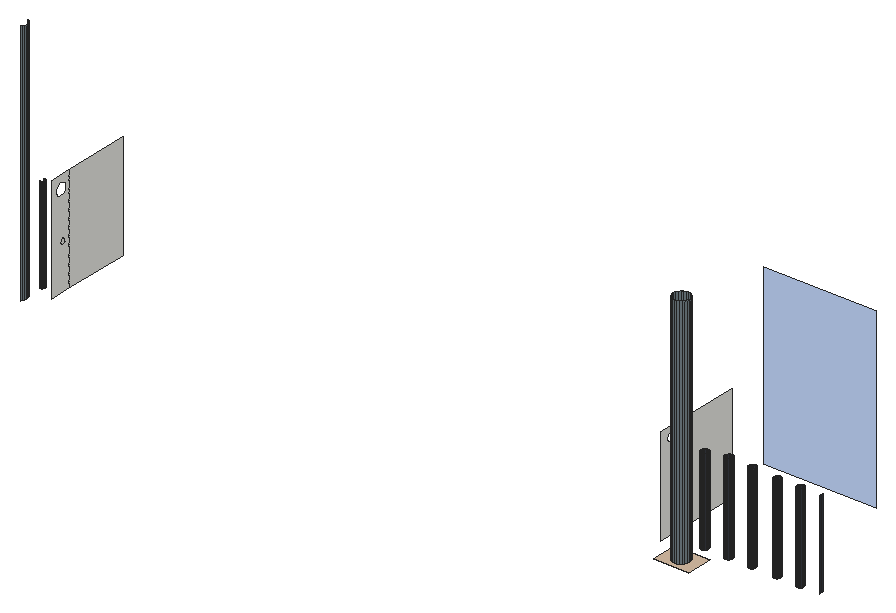
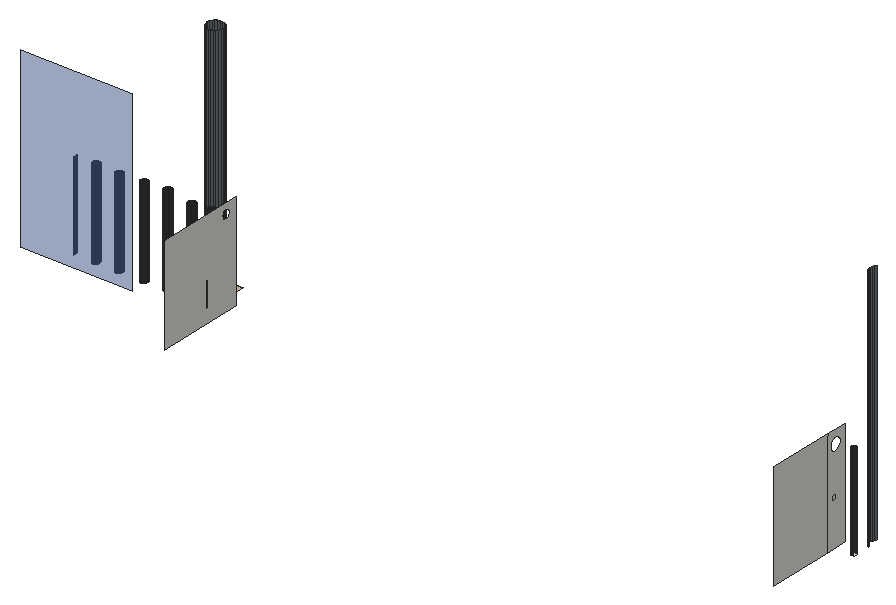
# SketchUp Ruby script. Lengths in inches.
U = 1.inch
M = Sketchup.active_model
def pt(a) = Geom::Point3d.new(a.map { |v| v * U })
def face(e, loops, mat)
  f = e.add_face(loops[0].map { |a| pt(a) })
  loops[1..].each { |l| e.add_face(l.map { |a| pt(a) }).erase! }
  f.material = f.back_material = mat if mat
  f
end
# faces: each face lists its corners as indices into pts; further lists are holes
def faces(e, pts, list, mat = nil) = list.each { |f| face(e, (f[0].is_a?(Array) ? f : [f]).map { |l| l.map { |i| pts[i] } }, mat) }
# xy, xz, yz: faces in a plane at the given z, y or x. An outline is a flat list of corners, or four numbers for a rectangle; further outlines are holes
def ring(l) = l.size == 4 ? [[l[0], l[1]], [l[2], l[1]], [l[2], l[3]], [l[0], l[3]]] : l.each_slice(2).to_a
def flat(e, list, mat, &to3) = list.each { |f| face(e, (f[0].is_a?(Array) ? f : [f]).map { |l| ring(l).map { |u, v| to3.(u, v) } }, mat) }
def xy(e, z, list, mat = nil) = flat(e, list, mat) { |x, y| [x, y, z] }
def xz(e, y, list, mat = nil) = flat(e, list, mat) { |x, z| [x, y, z] }
def yz(e, x, list, mat = nil) = flat(e, list, mat) { |y, z| [x, y, z] }
def lines(e, pts, list) = list.each { |a, b| e.add_line(pt(pts[a]), pt(pts[b])) }
# prism: a flat outline (further loops are holes) pulled along v
def prism(e, loops, v, mat = nil)
  f = face(e, loops, mat); d = Geom::Vector3d.new(v.map { |x| x * U })
  f.pushpull(f.normal.samedirection?(d) ? d.length : -d.length)
end
def box(e, o, s, mat = nil) = prism(e, [[o, [o[0] + s[0], o[1], o[2]], [o[0] + s[0], o[1] + s[1], o[2]], [o[0], o[1] + s[1], o[2]]]], [0, 0, s[2]], mat)
def at(x, y, z, deg = 0) = Geom::Transformation.translation(pt([x, y, z])) * Geom::Transformation.rotation(ORIGIN, Z_AXIS, deg.degrees)
def axes(o, x, y, z) = Geom::Transformation.new([*x, 0, *y, 0, *z, 0, *pt(o).to_a, 1])
def part(name) = M.definitions.add(name)
# library, detail: a bought-in or finely detailed component or shape, given as its bounding box
def library(name, o, s) = part(name).tap { |d| box(d.entities, o, s) }
def detail(e, o, s) = box(e.add_group.entities, o, s)
def put(e, d, t, mat = nil) = e.add_instance(d, t).tap { |i| i.material = mat if mat }
def group(e, t, mat = nil) = e.add_group.tap { |g| g.transformation = t; g.material = mat if mat }.entities
root = M.entities
M.materials.add("[Color M07]").color = [58, 58, 58]
M.materials.add("[Formica Laminate Dark]").color = [50, 53, 60]
M.materials.add("[Formica Laminate Light]").color = [213, 189, 164]
M.materials.add("[Formica Speckled Grey]").color = [112, 125, 132]
M.materials.add("[Translucent Glass Blue]").color = [85, 126, 201]
M.materials["[Translucent Glass Blue]"].alpha = 0.5
xy(root,272.93,[[302.73,84.01,302.14,84.08,301.6,84.31,301.14,84.67,300.78,85.13,300.55,85.67,300.48,86.26,300.55,86.84,300.78,87.38,301.14,87.85,301.6,88.21,302.14,88.43,302.73,88.51,303.31,88.43,303.85,88.21,304.32,87.85,304.67,87.38,304.9,86.84,304.98,86.26,304.9,85.67,304.67,85.13,304.32,84.67,303.85,84.31,303.31,84.08],[298.07,92.22,297.82,92.25,297.57,92.35,297.37,92.51,297.21,92.72,297.11,92.96,297.07,93.22,297.11,93.48,297.21,93.72,297.37,93.93,297.57,94.09,297.82,94.1875,298.07,94.22,298.33,94.1875,298.57,94.09,298.78,93.93,298.94,93.72,299.04,93.48,299.07,93.22,299.04,92.96,298.94,92.72,298.78,92.51,298.57,92.35,298.33,92.25],[303.57,92.22,303.32,92.25,303.07,92.35,302.87,92.51,302.71,92.72,302.61,92.96,302.57,93.22,302.61,93.48,302.71,93.72,302.87,93.93,303.07,94.09,303.32,94.1875,303.57,94.22,303.83,94.1875,304.07,94.09,304.28,93.93,304.44,93.72,304.54,93.48,304.57,93.22,304.54,92.96,304.44,92.72,304.28,92.51,304.07,92.35,303.83,92.25],[310.2,92.22,309.94,92.25,309.7,92.35,309.49,92.51,309.33,92.72,309.23,92.96,309.2,93.22,309.23,93.48,309.33,93.72,309.49,93.93,309.7,94.09,309.94,94.1875,310.2,94.22,310.46,94.1875,310.7,94.09,310.91,93.93,311.07,93.72,311.17,93.48,311.2,93.22,311.17,92.96,311.07,92.72,310.91,92.51,310.7,92.35,310.46,92.25],[316.7,92.22,316.44,92.25,316.2,92.35,315.99,92.51,315.83,92.72,315.73,92.96,315.7,93.22,315.73,93.48,315.83,93.72,315.99,93.93,316.2,94.09,316.44,94.1875,316.7,94.22,316.96,94.1875,317.2,94.09,317.41,93.93,317.57,93.72,317.67,93.48,317.7,93.22,317.67,92.96,317.57,92.72,317.41,92.51,317.2,92.35,316.96,92.25],
  [323.57,92.22,323.32,92.25,323.07,92.35,322.87,92.51,322.71,92.72,322.61,92.96,322.57,93.22,322.61,93.48,322.71,93.72,322.87,93.93,323.07,94.09,323.32,94.1875,323.57,94.22,323.83,94.1875,324.07,94.09,324.28,93.93,324.44,93.72,324.54,93.48,324.57,93.22,324.54,92.96,324.44,92.72,324.28,92.51,324.07,92.35,323.83,92.25],[329.95,92.22,329.69,92.25,329.45,92.35,329.24,92.51,329.08,92.72,328.98,92.96,328.95,93.22,328.98,93.48,329.08,93.72,329.24,93.93,329.45,94.09,329.69,94.1875,329.95,94.22,330.21,94.1875,330.45,94.09,330.66,93.93,330.82,93.72,330.92,93.48,330.95,93.22,330.92,92.96,330.82,92.72,330.66,92.51,330.45,92.35,330.21,92.25]])
xy(root,272.93,[[[298.18,82.54,307.63,89.73],[302.73,84.01,302.14,84.08,301.6,84.31,301.14,84.67,300.78,85.13,300.55,85.67,300.48,86.26,300.55,86.84,300.78,87.38,301.14,87.85,301.6,88.21,302.14,88.43,302.73,88.51,303.31,88.43,303.85,88.21,304.32,87.85,304.67,87.38,304.9,86.84,304.98,86.26,304.9,85.67,304.67,85.13,304.32,84.67,303.85,84.31,303.31,84.08]]],"[Formica Laminate Light]")
xy(root,273.71,[[121.84,91.87,121.66,91.89,121.5,91.96,121.36,92.07,121.25,92.21,121.18,92.38,121.15,92.56,121.18,92.73,121.25,92.9,121.36,93.04,121.5,93.15,121.66,93.22,121.84,93.24,122.02,93.22,122.1875,93.15,122.33,93.04,122.4375,92.9,122.51,92.73,122.53,92.56,122.51,92.38,122.4375,92.21,122.33,92.07,122.1875,91.96,122.02,91.89]])
xz(root,114.1,[[303.24,284.18,334.08,332.96]],"[Translucent Glass Blue]")
yz(root,126.66,[[[89.73,273.71,95.59,302.83],[92.96,297.54,93.42,297.6,93.84,297.77,94.2,298.05,94.48,298.41,94.65,298.84,94.71,299.29,94.65,299.74,94.48,300.16,94.2,300.53,93.84,300.8,93.42,300.98,92.96,301.04,92.51,300.98,92.09,300.8,91.73,300.53,91.45,300.16,91.27,299.74,91.21,299.29,91.27,298.84,91.45,298.41,91.73,298.05,92.09,297.77,92.51,297.6],[93.52,285.62,93.72,285.64,93.9,285.72,94.05,285.84,94.17,285.99,94.25,286.17,94.27,286.37,94.25,286.5625,94.17,286.74,94.05,286.9,93.9,287.02,93.72,287.09,93.52,287.12,93.33,287.09,93.15,287.02,92.99,286.9,92.875,286.74,92.8,286.5625,92.77,286.37,92.8,286.17,92.875,285.99,92.99,285.84,93.15,285.72,93.33,285.64]],[95.59,273.71,114.1,302.83],[93.52,285.62,93.72,285.64,93.9,285.72,94.05,285.84,94.17,285.99,94.25,286.17,94.27,286.37,94.25,286.5625,94.17,286.74,94.05,286.9,93.9,287.02,93.72,287.09,93.52,287.12,93.33,287.09,93.15,287.02,92.99,286.9,92.875,286.74,92.8,286.5625,92.77,286.37,92.8,286.17,92.875,285.99,92.99,285.84,93.15,285.72,93.33,285.64]])
yz(root,294.34,[[[89.73,272.93,114.1,299.8],[93.0625,295.87,92.74,295.91,92.4375,296.04,92.18,296.23,91.98,296.49,91.86,296.79,91.8125,297.12,91.86,297.44,91.98,297.74,92.18,298,92.4375,298.2,92.74,298.33,93.0625,298.37,93.39,298.33,93.6875,298.2,93.95,298,94.15,297.74,94.27,297.44,94.3125,297.12,94.27,296.79,94.15,296.49,93.95,296.23,93.6875,296.04,93.39,295.91]]])
p = [[302.14,84.08,272.93],[302.73,84.01,272.93],[302.73,84.01,337.71],[302.14,84.08,337.71],[303.31,84.08,272.93],[303.31,84.08,337.71],
  [301.6,84.31,272.93],[301.6,84.31,337.71],[303.85,84.31,272.93],[303.85,84.31,337.71],[301.14,84.67,272.93],[301.14,84.67,337.71],
  [304.32,84.67,272.93],[304.32,84.67,337.71],[300.78,85.13,272.93],[300.78,85.13,337.71],[304.67,85.13,272.93],[304.67,85.13,337.71],
  [300.55,85.67,272.93],[300.55,85.67,337.71],[304.9,85.67,272.93],[304.9,85.67,337.71],[300.48,86.26,272.93],[300.48,86.26,337.71],
  [304.98,86.26,272.93],[304.98,86.26,337.71],[300.55,86.84,272.93],[300.55,86.84,337.71],[304.9,86.84,272.93],[304.9,86.84,337.71],
  [300.78,87.38,272.93],[300.78,87.38,337.71],[304.67,87.38,272.93],[304.67,87.38,337.71],[301.14,87.85,272.93],[301.14,87.85,337.71],
  [304.32,87.85,272.93],[304.32,87.85,337.71],[301.6,88.21,272.93],[301.6,88.21,337.71],[303.85,88.21,272.93],[303.85,88.21,337.71],
  [302.14,88.43,272.93],[302.14,88.43,337.71],[303.31,88.43,272.93],[303.31,88.43,337.71],[302.73,88.51,272.93],[302.73,88.51,337.71],
  [297.82,92.25,272.93],[298.07,92.22,272.93],[298.07,92.22,297.05],[297.82,92.25,297.05],[298.33,92.25,272.93],[298.33,92.25,297.05],
  [303.32,92.25,272.93],[303.57,92.22,272.93],[303.57,92.22,296.68],[303.32,92.25,296.68],[303.83,92.25,272.93],[303.83,92.25,296.68],
  [309.94,92.25,272.93],[310.2,92.22,272.93],[310.2,92.22,297.74],[309.94,92.25,297.74],[310.46,92.25,272.93],[310.46,92.25,297.74],
  [316.44,92.25,272.93],[316.7,92.22,272.93],[316.7,92.22,297.44],[316.44,92.25,297.44],[316.96,92.25,272.93],[316.96,92.25,297.44],
  [323.32,92.25,272.93],[323.57,92.22,272.93],[323.57,92.22,297.05],[323.32,92.25,297.05],[323.83,92.25,272.93],[323.83,92.25,297.05],
  [329.69,92.25,272.93],[329.95,92.22,272.93],[329.95,92.22,297.18],[329.69,92.25,297.18],[330.21,92.25,272.93],[330.21,92.25,297.18],
  [297.57,92.35,272.93],[297.57,92.35,297.05],[298.57,92.35,272.93],[298.57,92.35,297.05],[303.07,92.35,272.93],[303.07,92.35,296.68],
  [304.07,92.35,272.93],[304.07,92.35,296.68],[309.7,92.35,272.93],[309.7,92.35,297.74],[310.7,92.35,272.93],[310.7,92.35,297.74],
  [316.2,92.35,272.93],[316.2,92.35,297.44],[317.2,92.35,272.93],[317.2,92.35,297.44],[323.07,92.35,272.93],[323.07,92.35,297.05],
  [324.07,92.35,272.93],[324.07,92.35,297.05],[329.45,92.35,272.93],[329.45,92.35,297.18],[330.45,92.35,272.93],[330.45,92.35,297.18],
  [297.37,92.51,272.93],[297.37,92.51,297.05],[298.78,92.51,272.93],[298.78,92.51,297.05],[302.87,92.51,272.93],[302.87,92.51,296.68],
  [304.28,92.51,272.93],[304.28,92.51,296.68],[309.49,92.51,272.93],[309.49,92.51,297.74],[310.91,92.51,272.93],[310.91,92.51,297.74],
  [315.99,92.51,272.93],[315.99,92.51,297.44],[317.41,92.51,272.93],[317.41,92.51,297.44],[322.87,92.51,272.93],[322.87,92.51,297.05],
  [324.28,92.51,272.93],[324.28,92.51,297.05],[329.24,92.51,272.93],[329.24,92.51,297.18],[330.66,92.51,272.93],[330.66,92.51,297.18],
  [297.21,92.72,272.93],[297.21,92.72,297.05],[298.94,92.72,272.93],[298.94,92.72,297.05],[302.71,92.72,272.93],[302.71,92.72,296.68],
  [304.44,92.72,272.93],[304.44,92.72,296.68],[309.33,92.72,272.93],[309.33,92.72,297.74],[311.07,92.72,272.93],[311.07,92.72,297.74],
  [315.83,92.72,272.93],[315.83,92.72,297.44],[317.57,92.72,272.93],[317.57,92.72,297.44],[322.71,92.72,272.93],[322.71,92.72,297.05],
  [324.44,92.72,272.93],[324.44,92.72,297.05],[329.08,92.72,272.93],[329.08,92.72,297.18],[330.82,92.72,272.93],[330.82,92.72,297.18],
  [297.11,92.96,272.93],[297.11,92.96,297.05],[299.04,92.96,272.93],[299.04,92.96,297.05],[302.61,92.96,272.93],[302.61,92.96,296.68],
  [304.54,92.96,272.93],[304.54,92.96,296.68],[309.23,92.96,272.93],[309.23,92.96,297.74],[311.17,92.96,272.93],[311.17,92.96,297.74],
  [315.73,92.96,272.93],[315.73,92.96,297.44],[317.67,92.96,272.93],[317.67,92.96,297.44],[322.61,92.96,272.93],[322.61,92.96,297.05],
  [324.54,92.96,272.93],[324.54,92.96,297.05],[328.98,92.96,272.93],[328.98,92.96,297.18],[330.92,92.96,272.93],[330.92,92.96,297.18],
  [335.48,93.39,272.93],[335.54,92.9375,272.93],[335.54,92.9375,297.11],[335.48,93.39,297.11],[297.07,93.22,272.93],[297.07,93.22,297.05],
  [299.07,93.22,272.93],[299.07,93.22,297.05],[302.57,93.22,272.93],[302.57,93.22,296.68],[304.57,93.22,272.93],[304.57,93.22,296.68],
  [309.2,93.22,272.93],[309.2,93.22,297.74],[311.2,93.22,272.93],[311.2,93.22,297.74],[315.7,93.22,272.93],[315.7,93.22,297.44],
  [317.7,93.22,272.93],[317.7,93.22,297.44],[322.57,93.22,272.93],[322.57,93.22,297.05],[324.57,93.22,272.93],[324.57,93.22,297.05],
  [328.95,93.22,272.93],[328.95,93.22,297.18],[330.95,93.22,272.93],[330.95,93.22,297.18],[297.11,93.48,272.93],[297.11,93.48,297.05],
  [299.04,93.48,272.93],[299.04,93.48,297.05],[302.61,93.48,272.93],[302.61,93.48,296.68],[304.54,93.48,272.93],[304.54,93.48,296.68],
  [309.23,93.48,272.93],[309.23,93.48,297.74],[311.17,93.48,272.93],[311.17,93.48,297.74],[315.73,93.48,272.93],[315.73,93.48,297.44],
  [317.67,93.48,272.93],[317.67,93.48,297.44],[322.61,93.48,272.93],[322.61,93.48,297.05],[324.54,93.48,272.93],[324.54,93.48,297.05],
  [328.98,93.48,272.93],[328.98,93.48,297.18],[330.92,93.48,272.93],[330.92,93.48,297.18],[335.54,93.84,272.93],[335.54,93.84,297.11],
  [297.21,93.72,272.93],[297.21,93.72,297.05],[298.94,93.72,272.93],[298.94,93.72,297.05],[302.71,93.72,272.93],[302.71,93.72,296.68],
  [304.44,93.72,272.93],[304.44,93.72,296.68],[309.33,93.72,272.93],[309.33,93.72,297.74],[311.07,93.72,272.93],[311.07,93.72,297.74],
  [315.83,93.72,272.93],[315.83,93.72,297.44],[317.57,93.72,272.93],[317.57,93.72,297.44],[322.71,93.72,272.93],[322.71,93.72,297.05],
  [324.44,93.72,272.93],[324.44,93.72,297.05],[329.08,93.72,272.93],[329.08,93.72,297.18],[330.82,93.72,272.93],[330.82,93.72,297.18],
  [297.37,93.93,272.93],[297.37,93.93,297.05],[298.78,93.93,272.93],[298.78,93.93,297.05],[302.87,93.93,272.93],[302.87,93.93,296.68],
  [304.28,93.93,272.93],[304.28,93.93,296.68],[309.49,93.93,272.93],[309.49,93.93,297.74],[310.91,93.93,272.93],[310.91,93.93,297.74],
  [315.99,93.93,272.93],[315.99,93.93,297.44],[317.41,93.93,272.93],[317.41,93.93,297.44],[322.87,93.93,272.93],[322.87,93.93,297.05],
  [324.28,93.93,272.93],[324.28,93.93,297.05],[329.24,93.93,272.93],[329.24,93.93,297.18],[330.66,93.93,272.93],[330.66,93.93,297.18],
  [297.57,94.09,272.93],[297.57,94.09,297.05],[298.57,94.09,272.93],[298.57,94.09,297.05],[303.07,94.09,272.93],[303.07,94.09,296.68],
  [304.07,94.09,272.93],[304.07,94.09,296.68],[309.7,94.09,272.93],[309.7,94.09,297.74],[310.7,94.09,272.93],[310.7,94.09,297.74],
  [316.2,94.09,272.93],[316.2,94.09,297.44],[317.2,94.09,272.93],[317.2,94.09,297.44],[323.07,94.09,272.93],[323.07,94.09,297.05],
  [324.07,94.09,272.93],[324.07,94.09,297.05],[329.45,94.09,272.93],[329.45,94.09,297.18],[330.45,94.09,272.93],[330.45,94.09,297.18],
  [297.82,94.1875,272.93],[297.82,94.1875,297.05],[298.33,94.1875,272.93],[298.33,94.1875,297.05],[303.32,94.1875,272.93],[303.32,94.1875,296.68],
  [303.83,94.1875,272.93],[303.83,94.1875,296.68],[309.94,94.1875,272.93],[309.85,94.15,297.74],[309.94,94.1875,297.74],[310.46,94.1875,272.93],
  [310.46,94.1875,297.74],[310.55,94.15,297.74],[316.44,94.1875,272.93],[316.44,94.1875,297.44],[316.96,94.1875,272.93],[316.96,94.1875,297.44],
  [323.32,94.1875,272.93],[323.32,94.1875,297.05],[323.83,94.1875,272.93],[323.83,94.1875,297.05],[329.69,94.1875,272.93],[329.69,94.1875,297.18],
  [330.21,94.1875,272.93],[330.21,94.1875,297.18],[298.07,94.22,272.93],[298.07,94.22,297.05],[303.57,94.22,272.93],[303.57,94.22,296.68],
  [310.2,94.22,272.93],[310.2,94.22,297.74],[316.7,94.22,272.93],[316.7,94.22,297.44],[323.57,94.22,272.93],[323.57,94.22,297.05],
  [329.95,94.22,272.93],[329.95,94.22,297.18],[121.86,84.89,273.71],[122.18,85.32,273.71],[122.18,85.32,341.31],[121.86,84.89,341.31],
  [122.39,85.82,273.71],[122.39,85.82,341.31],[122.46,86.35,273.71],[122.46,86.35,341.31],[122.39,86.89,273.71],[122.39,86.89,341.31],
  [122.18,87.38,273.71],[122.18,87.38,341.31],[121.86,87.8125,273.71],[121.86,87.8125,341.31],[121.43,88.14,273.71],[121.43,88.14,341.31],
  [121.66,91.89,273.71],[121.84,91.87,273.71],[121.84,91.87,299.96],[121.66,91.89,299.96],[122.02,91.89,273.71],[122.02,91.89,299.96],
  [122.1875,91.96,273.71],[122.1875,91.96,299.96],[122.33,92.07,273.71],[122.33,92.07,299.96],[122.4375,92.21,273.71],[122.4375,92.21,299.96],
  [122.51,92.38,273.71],[122.51,92.38,299.96],[122.53,92.56,273.71],[122.53,92.56,299.96],[122.51,92.73,273.71],[122.51,92.73,299.96],
  [122.4375,92.9,273.71],[122.4375,92.9,299.96],[122.33,93.04,273.71],[122.33,93.04,299.96],[122.1875,93.15,273.71],[122.1875,93.15,299.96],
  [121.84,93.24,273.71],[121.66,93.22,273.71],[121.66,93.22,299.96],[121.84,93.24,299.96],[122.02,93.22,273.71],[122.02,93.22,299.96]]
faces(root,p,[[0,1,2,3],[1,4,5,2],[6,0,3,7],[4,8,9,5],[10,6,7,11],[8,12,13,9],[14,10,11,15],[12,16,17,13],
  [18,14,15,19],[16,20,21,17],[22,18,19,23],[20,24,25,21],[26,22,23,27],[24,28,29,25],[30,26,27,31],[28,32,33,29],
  [34,30,31,35],[32,36,37,33],[38,34,35,39],[36,40,41,37],[42,38,39,43],[40,44,45,41],[46,42,43,47],[44,46,47,45],
  [344,345,346,347],[345,348,349,346],[348,350,351,349],[350,352,353,351],[352,354,355,353],[354,356,357,355],[356,358,359,357]],"[Formica Speckled Grey]")
faces(root,p,[[48,49,50,51],[49,52,53,50],[54,55,56,57],[55,58,59,56],[60,61,62,63],[61,64,65,62],[66,67,68,69],[67,70,71,68],
  [72,73,74,75],[73,76,77,74],[78,79,80,81],[79,82,83,80],[84,48,51,85],[52,86,87,53],[88,54,57,89],[58,90,91,59],
  [92,60,63,93],[64,94,95,65],[96,66,69,97],[70,98,99,71],[100,72,75,101],[76,102,103,77],[104,78,81,105],[82,106,107,83],
  [108,84,85,109],[86,110,111,87],[112,88,89,113],[90,114,115,91],[116,92,93,117],[94,118,119,95],[120,96,97,121],[98,122,123,99],
  [124,100,101,125],[102,126,127,103],[128,104,105,129],[106,130,131,107],[132,108,109,133],[110,134,135,111],[136,112,113,137],[114,138,139,115],
  [140,116,117,141],[118,142,143,119],[144,120,121,145],[122,146,147,123],[148,124,125,149],[126,150,151,127],[152,128,129,153],[130,154,155,131],
  [156,132,133,157],[134,158,159,135],[160,136,137,161],[138,162,163,139],[164,140,141,165],[142,166,167,143],[168,144,145,169],[146,170,171,147],
  [172,148,149,173],[150,174,175,151],[176,152,153,177],[154,178,179,155],[180,181,182,183],[184,156,157,185],[158,186,187,159],[188,160,161,189],
  [162,190,191,163],[192,164,165,193],[166,194,195,167],[196,168,169,197],[170,198,199,171],[200,172,173,201],[174,202,203,175],[204,176,177,205],
  [178,206,207,179],[208,184,185,209],[186,210,211,187],[212,188,189,213],[190,214,215,191],[216,192,193,217],[194,218,219,195],[220,196,197,221],
  [198,222,223,199],[224,200,201,225],[202,226,227,203],[228,204,205,229],[206,230,231,207],[232,180,183,233],[234,208,209,235],[210,236,237,211],
  [238,212,213,239],[214,240,241,215],[242,216,217,243],[218,244,245,219],[246,220,221,247],[222,248,249,223],[250,224,225,251],[226,252,253,227],
  [254,228,229,255],[230,256,257,231],[258,234,235,259],[236,260,261,237],[262,238,239,263],[240,264,265,241],[266,242,243,267],[244,268,269,245],
  [270,246,247,271],[248,272,273,249],[274,250,251,275],[252,276,277,253],[278,254,255,279],[256,280,281,257],[282,258,259,283],[260,284,285,261],
  [286,262,263,287],[264,288,289,265],[290,266,267,291],[268,292,293,269],[294,270,271,295],[272,296,297,273],[298,274,275,299],[276,300,301,277],
  [302,278,279,303],[280,304,305,281],[306,282,283,307],[284,308,309,285],[310,286,287,311],[288,312,313,289],[314,290,291,315,316],[292,317,318,319,293],
  [320,294,295,321],[296,322,323,297],[324,298,299,325],[300,326,327,301],[328,302,303,329],[304,330,331,305],[332,306,307,333],[308,332,333,309],
  [334,310,311,335],[312,334,335,313],[336,314,316,337],[317,336,337,318],[338,320,321,339],[322,338,339,323],[340,324,325,341],[326,340,341,327],
  [342,328,329,343],[330,342,343,331]],"[Formica Laminate Dark]")
faces(root,p,[[360,361,362,363],[361,364,365,362],[364,366,367,365],[366,368,369,367],[368,370,371,369],[370,372,373,371],[372,374,375,373],[374,376,377,375],
  [376,378,379,377],[378,380,381,379],[380,382,383,381],[384,385,386,387],[388,384,387,389],[382,388,389,383]],"[Color M07]")
